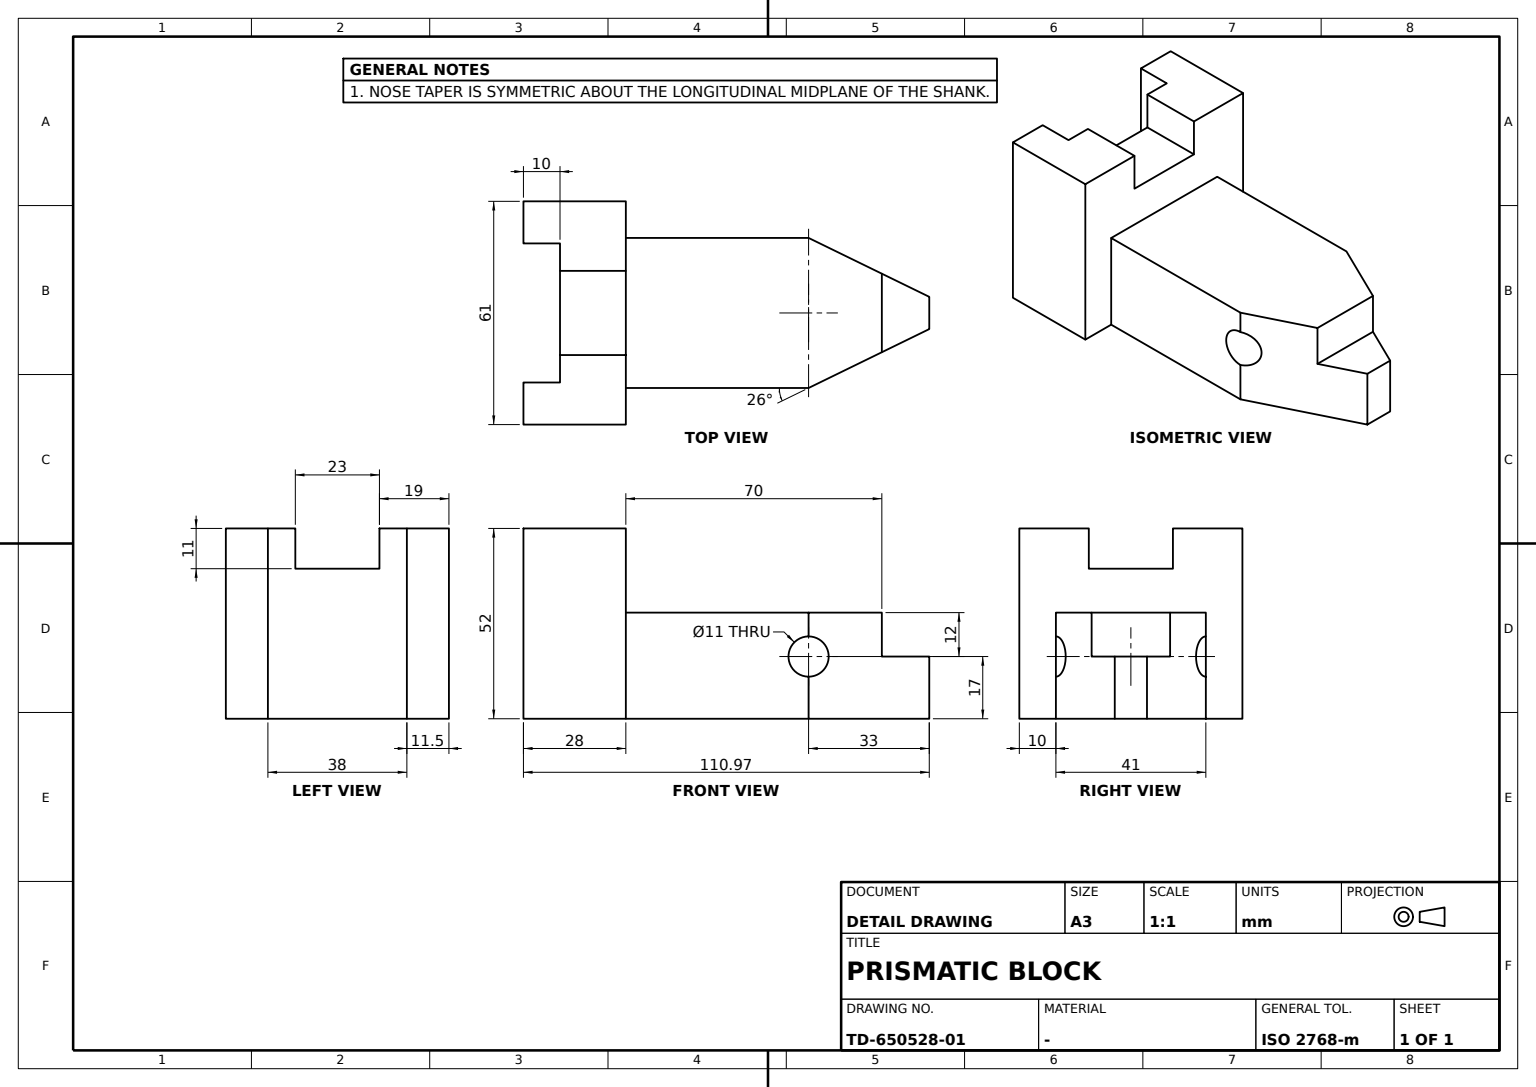
ISO-10303-21;
HEADER;
FILE_DESCRIPTION((''),'2;1');
FILE_NAME('','',(''),(''),'','','');
FILE_SCHEMA(('AUTOMOTIVE_DESIGN'));
ENDSEC;
DATA;
#1=APPLICATION_CONTEXT('');
#2=PRODUCT_CONTEXT('',#1,'mechanical');
#3=PRODUCT('','','',(#2));
#4=PRODUCT_DEFINITION_FORMATION('','',#3);
#5=PRODUCT_DEFINITION_CONTEXT('',#1,'design');
#6=PRODUCT_DEFINITION('','',#4,#5);
#7=PRODUCT_DEFINITION_SHAPE('','',#6);
#8=(LENGTH_UNIT()NAMED_UNIT(*)SI_UNIT(.MILLI.,.METRE.));
#9=(NAMED_UNIT(*)PLANE_ANGLE_UNIT()SI_UNIT($,.RADIAN.));
#10=(NAMED_UNIT(*)SI_UNIT($,.STERADIAN.)SOLID_ANGLE_UNIT());
#11=UNCERTAINTY_MEASURE_WITH_UNIT(LENGTH_MEASURE(0.005),#8,'distance_accuracy_value','');
#12=(GEOMETRIC_REPRESENTATION_CONTEXT(3)GLOBAL_UNCERTAINTY_ASSIGNED_CONTEXT((#11))GLOBAL_UNIT_ASSIGNED_CONTEXT((#8,#9,#10))REPRESENTATION_CONTEXT('',''));
#13=CARTESIAN_POINT('',(100.968771,-4.404825,0.));
#14=VERTEX_POINT('',#13);
#15=CARTESIAN_POINT('',(100.968771,4.404825,0.));
#16=VERTEX_POINT('',#15);
#17=DIRECTION('',(0.,1.,0.));
#18=VECTOR('',#17,1000.);
#19=LINE('',#13,#18);
#20=EDGE_CURVE('',#14,#16,#19,.T.);
#21=ORIENTED_EDGE('',*,*,#20,.T.);
#22=CARTESIAN_POINT('',(100.968771,4.404825,17.));
#23=VERTEX_POINT('',#22);
#24=DIRECTION('',(0.,0.,1.));
#25=VECTOR('',#24,1000.);
#26=LINE('',#15,#25);
#27=EDGE_CURVE('',#16,#23,#26,.T.);
#28=ORIENTED_EDGE('',*,*,#27,.T.);
#29=CARTESIAN_POINT('',(100.968771,-4.404825,17.));
#30=VERTEX_POINT('',#29);
#31=LINE('',#29,#18);
#32=EDGE_CURVE('',#30,#23,#31,.T.);
#33=ORIENTED_EDGE('',*,*,#32,.F.);
#34=LINE('',#13,#25);
#35=EDGE_CURVE('',#14,#30,#34,.T.);
#36=ORIENTED_EDGE('',*,*,#35,.F.);
#37=EDGE_LOOP('',(#21,#28,#33,#36));
#38=FACE_BOUND('',#37,.T.);
#39=DIRECTION('',(1.,0.,0.));
#40=DIRECTION('',(0.,0.,-1.));
#41=AXIS2_PLACEMENT_3D('',#13,#39,#40);
#42=PLANE('',#41);
#43=ADVANCED_FACE('',(#38),#42,.T.);
#44=CARTESIAN_POINT('',(-10.,-19.,0.));
#45=VERTEX_POINT('',#44);
#46=CARTESIAN_POINT('',(-10.,-30.5,0.));
#47=VERTEX_POINT('',#46);
#48=DIRECTION('',(0.,-1.,0.));
#49=VECTOR('',#48,1000.);
#50=LINE('',#44,#49);
#51=EDGE_CURVE('',#45,#47,#50,.T.);
#52=ORIENTED_EDGE('',*,*,#51,.T.);
#53=CARTESIAN_POINT('',(-10.,-30.5,52.));
#54=VERTEX_POINT('',#53);
#55=LINE('',#46,#25);
#56=EDGE_CURVE('',#47,#54,#55,.T.);
#57=ORIENTED_EDGE('',*,*,#56,.T.);
#58=CARTESIAN_POINT('',(-10.,-19.,52.));
#59=VERTEX_POINT('',#58);
#60=LINE('',#58,#49);
#61=EDGE_CURVE('',#59,#54,#60,.T.);
#62=ORIENTED_EDGE('',*,*,#61,.F.);
#63=LINE('',#44,#25);
#64=EDGE_CURVE('',#45,#59,#63,.T.);
#65=ORIENTED_EDGE('',*,*,#64,.F.);
#66=EDGE_LOOP('',(#52,#57,#62,#65));
#67=FACE_BOUND('',#66,.T.);
#68=DIRECTION('',(-1.,0.,0.));
#69=AXIS2_PLACEMENT_3D('',#44,#68,#48);
#70=PLANE('',#69);
#71=ADVANCED_FACE('',(#67),#70,.T.);
#72=CARTESIAN_POINT('',(0.,19.,0.));
#73=VERTEX_POINT('',#72);
#74=CARTESIAN_POINT('',(0.,19.,52.));
#75=VERTEX_POINT('',#74);
#76=LINE('',#72,#25);
#77=EDGE_CURVE('',#73,#75,#76,.T.);
#78=ORIENTED_EDGE('',*,*,#77,.T.);
#79=CARTESIAN_POINT('',(-10.,19.,52.));
#80=VERTEX_POINT('',#79);
#81=VECTOR('',#39,1000.);
#82=LINE('',#79,#81);
#83=EDGE_CURVE('',#80,#75,#82,.T.);
#84=ORIENTED_EDGE('',*,*,#83,.F.);
#85=CARTESIAN_POINT('',(-10.,19.,0.));
#86=VERTEX_POINT('',#85);
#87=LINE('',#85,#25);
#88=EDGE_CURVE('',#86,#80,#87,.T.);
#89=ORIENTED_EDGE('',*,*,#88,.F.);
#90=LINE('',#85,#81);
#91=EDGE_CURVE('',#86,#73,#90,.T.);
#92=ORIENTED_EDGE('',*,*,#91,.T.);
#93=EDGE_LOOP('',(#78,#84,#89,#92));
#94=FACE_BOUND('',#93,.T.);
#95=AXIS2_PLACEMENT_3D('',#85,#48,#40);
#96=PLANE('',#95);
#97=ADVANCED_FACE('',(#94),#96,.T.);
#98=ORIENTED_EDGE('',*,*,#64,.T.);
#99=CARTESIAN_POINT('',(0.,-19.,52.));
#100=VERTEX_POINT('',#99);
#101=VECTOR('',#68,1000.);
#102=LINE('',#99,#101);
#103=EDGE_CURVE('',#100,#59,#102,.T.);
#104=ORIENTED_EDGE('',*,*,#103,.F.);
#105=CARTESIAN_POINT('',(0.,-19.,0.));
#106=VERTEX_POINT('',#105);
#107=LINE('',#105,#25);
#108=EDGE_CURVE('',#106,#100,#107,.T.);
#109=ORIENTED_EDGE('',*,*,#108,.F.);
#110=LINE('',#105,#101);
#111=EDGE_CURVE('',#106,#45,#110,.T.);
#112=ORIENTED_EDGE('',*,*,#111,.T.);
#113=EDGE_LOOP('',(#98,#104,#109,#112));
#114=FACE_BOUND('',#113,.T.);
#115=AXIS2_PLACEMENT_3D('',#105,#17,#24);
#116=PLANE('',#115);
#117=ADVANCED_FACE('',(#114),#116,.T.);
#118=CARTESIAN_POINT('',(-10.,30.5,0.));
#119=VERTEX_POINT('',#118);
#120=LINE('',#118,#49);
#121=EDGE_CURVE('',#119,#86,#120,.T.);
#122=ORIENTED_EDGE('',*,*,#121,.T.);
#123=ORIENTED_EDGE('',*,*,#88,.T.);
#124=CARTESIAN_POINT('',(-10.,30.5,52.));
#125=VERTEX_POINT('',#124);
#126=LINE('',#124,#49);
#127=EDGE_CURVE('',#125,#80,#126,.T.);
#128=ORIENTED_EDGE('',*,*,#127,.F.);
#129=LINE('',#118,#25);
#130=EDGE_CURVE('',#119,#125,#129,.T.);
#131=ORIENTED_EDGE('',*,*,#130,.F.);
#132=EDGE_LOOP('',(#122,#123,#128,#131));
#133=FACE_BOUND('',#132,.T.);
#134=AXIS2_PLACEMENT_3D('',#118,#68,#24);
#135=PLANE('',#134);
#136=ADVANCED_FACE('',(#133),#135,.T.);
#137=CARTESIAN_POINT('',(18.,20.5,0.));
#138=VERTEX_POINT('',#137);
#139=CARTESIAN_POINT('',(18.,20.5,29.));
#140=VERTEX_POINT('',#139);
#141=LINE('',#137,#25);
#142=EDGE_CURVE('',#138,#140,#141,.T.);
#143=ORIENTED_EDGE('',*,*,#142,.F.);
#144=CARTESIAN_POINT('',(18.,30.5,0.));
#145=VERTEX_POINT('',#144);
#146=CARTESIAN_POINT('',(18.,-30.5,0.));
#147=LINE('',#146,#18);
#148=EDGE_CURVE('',#138,#145,#147,.T.);
#149=ORIENTED_EDGE('',*,*,#148,.T.);
#150=CARTESIAN_POINT('',(18.,30.5,52.));
#151=VERTEX_POINT('',#150);
#152=LINE('',#144,#25);
#153=EDGE_CURVE('',#145,#151,#152,.T.);
#154=ORIENTED_EDGE('',*,*,#153,.T.);
#155=CARTESIAN_POINT('',(18.,11.5,52.));
#156=VERTEX_POINT('',#155);
#157=CARTESIAN_POINT('',(18.,0.,52.));
#158=LINE('',#157,#18);
#159=EDGE_CURVE('',#156,#151,#158,.T.);
#160=ORIENTED_EDGE('',*,*,#159,.F.);
#161=CARTESIAN_POINT('',(18.,11.5,41.));
#162=VERTEX_POINT('',#161);
#163=VECTOR('',#40,1000.);
#164=LINE('',#155,#163);
#165=EDGE_CURVE('',#156,#162,#164,.T.);
#166=ORIENTED_EDGE('',*,*,#165,.T.);
#167=CARTESIAN_POINT('',(18.,-11.5,41.));
#168=VERTEX_POINT('',#167);
#169=LINE('',#167,#18);
#170=EDGE_CURVE('',#168,#162,#169,.T.);
#171=ORIENTED_EDGE('',*,*,#170,.F.);
#172=CARTESIAN_POINT('',(18.,-11.5,52.));
#173=VERTEX_POINT('',#172);
#174=LINE('',#172,#163);
#175=EDGE_CURVE('',#173,#168,#174,.T.);
#176=ORIENTED_EDGE('',*,*,#175,.F.);
#177=CARTESIAN_POINT('',(18.,-30.5,52.));
#178=VERTEX_POINT('',#177);
#179=EDGE_CURVE('',#178,#173,#158,.T.);
#180=ORIENTED_EDGE('',*,*,#179,.F.);
#181=VERTEX_POINT('',#146);
#182=LINE('',#146,#25);
#183=EDGE_CURVE('',#181,#178,#182,.T.);
#184=ORIENTED_EDGE('',*,*,#183,.F.);
#185=CARTESIAN_POINT('',(18.,-20.5,0.));
#186=VERTEX_POINT('',#185);
#187=EDGE_CURVE('',#181,#186,#147,.T.);
#188=ORIENTED_EDGE('',*,*,#187,.T.);
#189=CARTESIAN_POINT('',(18.,-20.5,29.));
#190=VERTEX_POINT('',#189);
#191=LINE('',#185,#25);
#192=EDGE_CURVE('',#186,#190,#191,.T.);
#193=ORIENTED_EDGE('',*,*,#192,.T.);
#194=LINE('',#139,#49);
#195=EDGE_CURVE('',#140,#190,#194,.T.);
#196=ORIENTED_EDGE('',*,*,#195,.F.);
#197=EDGE_LOOP('',(#143,#149,#154,#160,#166,#171,#176,#180,#184,#188,#193,#196));
#198=FACE_BOUND('',#197,.T.);
#199=CARTESIAN_POINT('',(18.,0.,0.));
#200=AXIS2_PLACEMENT_3D('',#199,#39,#40);
#201=PLANE('',#200);
#202=ADVANCED_FACE('',(#198),#201,.T.);
#203=CARTESIAN_POINT('',(0.,11.5,52.));
#204=VERTEX_POINT('',#203);
#205=CARTESIAN_POINT('',(0.,0.,52.));
#206=LINE('',#205,#49);
#207=EDGE_CURVE('',#75,#204,#206,.T.);
#208=ORIENTED_EDGE('',*,*,#207,.F.);
#209=ORIENTED_EDGE('',*,*,#77,.F.);
#210=LINE('',#72,#49);
#211=EDGE_CURVE('',#73,#106,#210,.T.);
#212=ORIENTED_EDGE('',*,*,#211,.T.);
#213=ORIENTED_EDGE('',*,*,#108,.T.);
#214=CARTESIAN_POINT('',(0.,-11.5,52.));
#215=VERTEX_POINT('',#214);
#216=EDGE_CURVE('',#215,#100,#206,.T.);
#217=ORIENTED_EDGE('',*,*,#216,.F.);
#218=CARTESIAN_POINT('',(0.,-11.5,41.));
#219=VERTEX_POINT('',#218);
#220=LINE('',#214,#163);
#221=EDGE_CURVE('',#215,#219,#220,.T.);
#222=ORIENTED_EDGE('',*,*,#221,.T.);
#223=CARTESIAN_POINT('',(0.,11.5,41.));
#224=VERTEX_POINT('',#223);
#225=LINE('',#223,#49);
#226=EDGE_CURVE('',#224,#219,#225,.T.);
#227=ORIENTED_EDGE('',*,*,#226,.F.);
#228=LINE('',#203,#163);
#229=EDGE_CURVE('',#204,#224,#228,.T.);
#230=ORIENTED_EDGE('',*,*,#229,.F.);
#231=EDGE_LOOP('',(#208,#209,#212,#213,#217,#222,#227,#230));
#232=FACE_BOUND('',#231,.T.);
#233=CARTESIAN_POINT('',(0.,0.,0.));
#234=AXIS2_PLACEMENT_3D('',#233,#68,#48);
#235=PLANE('',#234);
#236=ADVANCED_FACE('',(#232),#235,.T.);
#237=CARTESIAN_POINT('',(67.968771,-20.5,22.5));
#238=VERTEX_POINT('',#237);
#239=CARTESIAN_POINT('',(67.968771,20.5,22.5));
#240=VERTEX_POINT('',#239);
#241=CARTESIAN_POINT('',(67.968771,-30.,22.5));
#242=LINE('',#241,#18);
#243=EDGE_CURVE('',#238,#240,#242,.T.);
#244=ORIENTED_EDGE('',*,*,#243,.F.);
#245=CARTESIAN_POINT('',(67.968771,-20.5,11.5));
#246=VERTEX_POINT('',#245);
#247=CARTESIAN_POINT('',(67.968771,-20.5,17.));
#248=AXIS2_PLACEMENT_3D('',#247,#17,#39);
#249=CIRCLE('',#248,5.5);
#250=EDGE_CURVE('',#246,#238,#249,.T.);
#251=ORIENTED_EDGE('',*,*,#250,.F.);
#252=CARTESIAN_POINT('',(67.968771,20.5,11.5));
#253=VERTEX_POINT('',#252);
#254=CARTESIAN_POINT('',(67.968771,-30.,11.5));
#255=LINE('',#254,#18);
#256=EDGE_CURVE('',#253,#246,#255,.F.);
#257=ORIENTED_EDGE('',*,*,#256,.F.);
#258=CARTESIAN_POINT('',(67.968771,20.5,17.));
#259=AXIS2_PLACEMENT_3D('',#258,#48,#68);
#260=CIRCLE('',#259,5.5);
#261=EDGE_CURVE('',#240,#253,#260,.T.);
#262=ORIENTED_EDGE('',*,*,#261,.F.);
#263=EDGE_LOOP('',(#244,#251,#257,#262));
#264=FACE_BOUND('',#263,.T.);
#265=CARTESIAN_POINT('',(67.968771,-30.,17.));
#266=AXIS2_PLACEMENT_3D('',#265,#17,#24);
#267=CYLINDRICAL_SURFACE('',#266,5.5);
#268=ADVANCED_FACE('',(#264),#267,.F.);
#269=LINE('',#53,#81);
#270=EDGE_CURVE('',#54,#178,#269,.T.);
#271=ORIENTED_EDGE('',*,*,#270,.T.);
#272=ORIENTED_EDGE('',*,*,#179,.T.);
#273=LINE('',#214,#81);
#274=EDGE_CURVE('',#215,#173,#273,.T.);
#275=ORIENTED_EDGE('',*,*,#274,.F.);
#276=ORIENTED_EDGE('',*,*,#216,.T.);
#277=ORIENTED_EDGE('',*,*,#103,.T.);
#278=ORIENTED_EDGE('',*,*,#61,.T.);
#279=EDGE_LOOP('',(#271,#272,#275,#276,#277,#278));
#280=FACE_BOUND('',#279,.T.);
#281=AXIS2_PLACEMENT_3D('',#205,#24,#39);
#282=PLANE('',#281);
#283=ADVANCED_FACE('',(#280),#282,.T.);
#284=CARTESIAN_POINT('',(88.,-10.730117,29.));
#285=VERTEX_POINT('',#284);
#286=CARTESIAN_POINT('',(88.,-10.730117,17.));
#287=VERTEX_POINT('',#286);
#288=LINE('',#284,#163);
#289=EDGE_CURVE('',#285,#287,#288,.T.);
#290=ORIENTED_EDGE('',*,*,#289,.T.);
#291=CARTESIAN_POINT('',(88.,10.730117,17.));
#292=VERTEX_POINT('',#291);
#293=LINE('',#291,#18);
#294=EDGE_CURVE('',#287,#292,#293,.T.);
#295=ORIENTED_EDGE('',*,*,#294,.T.);
#296=CARTESIAN_POINT('',(88.,10.730117,29.));
#297=VERTEX_POINT('',#296);
#298=LINE('',#296,#163);
#299=EDGE_CURVE('',#297,#292,#298,.T.);
#300=ORIENTED_EDGE('',*,*,#299,.F.);
#301=LINE('',#296,#49);
#302=EDGE_CURVE('',#297,#285,#301,.T.);
#303=ORIENTED_EDGE('',*,*,#302,.T.);
#304=EDGE_LOOP('',(#290,#295,#300,#303));
#305=FACE_BOUND('',#304,.T.);
#306=AXIS2_PLACEMENT_3D('',#296,#39,#17);
#307=PLANE('',#306);
#308=ADVANCED_FACE('',(#305),#307,.T.);
#309=ORIENTED_EDGE('',*,*,#187,.F.);
#310=LINE('',#46,#81);
#311=EDGE_CURVE('',#47,#181,#310,.T.);
#312=ORIENTED_EDGE('',*,*,#311,.F.);
#313=ORIENTED_EDGE('',*,*,#51,.F.);
#314=ORIENTED_EDGE('',*,*,#111,.F.);
#315=ORIENTED_EDGE('',*,*,#211,.F.);
#316=ORIENTED_EDGE('',*,*,#91,.F.);
#317=ORIENTED_EDGE('',*,*,#121,.F.);
#318=LINE('',#144,#101);
#319=EDGE_CURVE('',#145,#119,#318,.T.);
#320=ORIENTED_EDGE('',*,*,#319,.F.);
#321=ORIENTED_EDGE('',*,*,#148,.F.);
#322=CARTESIAN_POINT('',(67.968771,20.5,0.));
#323=VERTEX_POINT('',#322);
#324=LINE('',#322,#101);
#325=EDGE_CURVE('',#323,#138,#324,.T.);
#326=ORIENTED_EDGE('',*,*,#325,.F.);
#327=DIRECTION('',(-0.898794046,0.438371147,0.));
#328=VECTOR('',#327,1000.);
#329=LINE('',#15,#328);
#330=EDGE_CURVE('',#16,#323,#329,.T.);
#331=ORIENTED_EDGE('',*,*,#330,.F.);
#332=ORIENTED_EDGE('',*,*,#20,.F.);
#333=CARTESIAN_POINT('',(67.968771,-20.5,0.));
#334=VERTEX_POINT('',#333);
#335=DIRECTION('',(0.898794046,0.438371147,0.));
#336=VECTOR('',#335,1000.);
#337=LINE('',#333,#336);
#338=EDGE_CURVE('',#334,#14,#337,.T.);
#339=ORIENTED_EDGE('',*,*,#338,.F.);
#340=LINE('',#185,#81);
#341=EDGE_CURVE('',#186,#334,#340,.T.);
#342=ORIENTED_EDGE('',*,*,#341,.F.);
#343=EDGE_LOOP('',(#309,#312,#313,#314,#315,#316,#317,#320,#321,#326,#331,#332,#339,#342));
#344=FACE_BOUND('',#343,.T.);
#345=AXIS2_PLACEMENT_3D('',#233,#24,#39);
#346=PLANE('',#345);
#347=ADVANCED_FACE('',(#344),#346,.F.);
#348=ORIENTED_EDGE('',*,*,#229,.T.);
#349=LINE('',#161,#81);
#350=EDGE_CURVE('',#224,#162,#349,.T.);
#351=ORIENTED_EDGE('',*,*,#350,.T.);
#352=ORIENTED_EDGE('',*,*,#165,.F.);
#353=LINE('',#155,#101);
#354=EDGE_CURVE('',#156,#204,#353,.T.);
#355=ORIENTED_EDGE('',*,*,#354,.T.);
#356=EDGE_LOOP('',(#348,#351,#352,#355));
#357=FACE_BOUND('',#356,.T.);
#358=AXIS2_PLACEMENT_3D('',#155,#48,#39);
#359=PLANE('',#358);
#360=ADVANCED_FACE('',(#357),#359,.T.);
#361=ORIENTED_EDGE('',*,*,#243,.T.);
#362=CARTESIAN_POINT('',(78.968771,15.134942,11.5));
#363=CARTESIAN_POINT('',(78.968771,15.134942,22.5));
#364=(BOUNDED_CURVE()B_SPLINE_CURVE(3,(#252,#362,#363,#239),.UNSPECIFIED.,.F.,.F.)B_SPLINE_CURVE_WITH_KNOTS((4,4),(1.570796327,4.71238898),.UNSPECIFIED.)CURVE()GEOMETRIC_REPRESENTATION_ITEM()RATIONAL_B_SPLINE_CURVE((1.,0.333333333,0.333333333,1.))REPRESENTATION_ITEM(''));
#365=EDGE_CURVE('',#253,#240,#364,.T.);
#366=ORIENTED_EDGE('',*,*,#365,.F.);
#367=ORIENTED_EDGE('',*,*,#256,.T.);
#368=CARTESIAN_POINT('',(78.968771,-15.134942,22.5));
#369=CARTESIAN_POINT('',(78.968771,-15.134942,11.5));
#370=(BOUNDED_CURVE()B_SPLINE_CURVE(3,(#237,#368,#369,#245),.UNSPECIFIED.,.F.,.F.)B_SPLINE_CURVE_WITH_KNOTS((4,4),(4.71238898,7.853981634),.UNSPECIFIED.)CURVE()GEOMETRIC_REPRESENTATION_ITEM()RATIONAL_B_SPLINE_CURVE((1.,0.333333333,0.333333333,1.))REPRESENTATION_ITEM(''));
#371=EDGE_CURVE('',#238,#246,#370,.T.);
#372=ORIENTED_EDGE('',*,*,#371,.F.);
#373=EDGE_LOOP('',(#361,#366,#367,#372));
#374=FACE_BOUND('',#373,.T.);
#375=ADVANCED_FACE('',(#374),#267,.F.);
#376=CARTESIAN_POINT('',(67.968771,20.5,29.));
#377=VERTEX_POINT('',#376);
#378=LINE('',#376,#101);
#379=EDGE_CURVE('',#377,#140,#378,.T.);
#380=ORIENTED_EDGE('',*,*,#379,.T.);
#381=ORIENTED_EDGE('',*,*,#195,.T.);
#382=CARTESIAN_POINT('',(67.968771,-20.5,29.));
#383=VERTEX_POINT('',#382);
#384=LINE('',#189,#81);
#385=EDGE_CURVE('',#190,#383,#384,.T.);
#386=ORIENTED_EDGE('',*,*,#385,.T.);
#387=LINE('',#382,#336);
#388=EDGE_CURVE('',#383,#285,#387,.T.);
#389=ORIENTED_EDGE('',*,*,#388,.T.);
#390=ORIENTED_EDGE('',*,*,#302,.F.);
#391=CARTESIAN_POINT('',(100.968771,4.404825,29.));
#392=LINE('',#391,#328);
#393=EDGE_CURVE('',#297,#377,#392,.T.);
#394=ORIENTED_EDGE('',*,*,#393,.T.);
#395=EDGE_LOOP('',(#380,#381,#386,#389,#390,#394));
#396=FACE_BOUND('',#395,.T.);
#397=CARTESIAN_POINT('',(0.,0.,29.));
#398=AXIS2_PLACEMENT_3D('',#397,#24,#39);
#399=PLANE('',#398);
#400=ADVANCED_FACE('',(#396),#399,.T.);
#401=ORIENTED_EDGE('',*,*,#175,.T.);
#402=LINE('',#218,#101);
#403=EDGE_CURVE('',#168,#219,#402,.T.);
#404=ORIENTED_EDGE('',*,*,#403,.T.);
#405=ORIENTED_EDGE('',*,*,#221,.F.);
#406=ORIENTED_EDGE('',*,*,#274,.T.);
#407=EDGE_LOOP('',(#401,#404,#405,#406));
#408=FACE_BOUND('',#407,.T.);
#409=AXIS2_PLACEMENT_3D('',#214,#17,#68);
#410=PLANE('',#409);
#411=ADVANCED_FACE('',(#408),#410,.T.);
#412=ORIENTED_EDGE('',*,*,#226,.T.);
#413=ORIENTED_EDGE('',*,*,#403,.F.);
#414=ORIENTED_EDGE('',*,*,#170,.T.);
#415=ORIENTED_EDGE('',*,*,#350,.F.);
#416=EDGE_LOOP('',(#412,#413,#414,#415));
#417=FACE_BOUND('',#416,.T.);
#418=CARTESIAN_POINT('',(0.,0.,41.));
#419=AXIS2_PLACEMENT_3D('',#418,#24,#39);
#420=PLANE('',#419);
#421=ADVANCED_FACE('',(#417),#420,.T.);
#422=LINE('',#333,#25);
#423=EDGE_CURVE('',#238,#383,#422,.T.);
#424=ORIENTED_EDGE('',*,*,#423,.T.);
#425=ORIENTED_EDGE('',*,*,#385,.F.);
#426=ORIENTED_EDGE('',*,*,#192,.F.);
#427=ORIENTED_EDGE('',*,*,#341,.T.);
#428=EDGE_CURVE('',#334,#246,#422,.T.);
#429=ORIENTED_EDGE('',*,*,#428,.T.);
#430=ORIENTED_EDGE('',*,*,#250,.T.);
#431=EDGE_LOOP('',(#424,#425,#426,#427,#429,#430));
#432=FACE_BOUND('',#431,.T.);
#433=AXIS2_PLACEMENT_3D('',#185,#48,#39);
#434=PLANE('',#433);
#435=ADVANCED_FACE('',(#432),#434,.T.);
#436=ORIENTED_EDGE('',*,*,#159,.T.);
#437=LINE('',#150,#101);
#438=EDGE_CURVE('',#151,#125,#437,.T.);
#439=ORIENTED_EDGE('',*,*,#438,.T.);
#440=ORIENTED_EDGE('',*,*,#127,.T.);
#441=ORIENTED_EDGE('',*,*,#83,.T.);
#442=ORIENTED_EDGE('',*,*,#207,.T.);
#443=ORIENTED_EDGE('',*,*,#354,.F.);
#444=EDGE_LOOP('',(#436,#439,#440,#441,#442,#443));
#445=FACE_BOUND('',#444,.T.);
#446=ADVANCED_FACE('',(#445),#282,.T.);
#447=ORIENTED_EDGE('',*,*,#27,.F.);
#448=ORIENTED_EDGE('',*,*,#330,.T.);
#449=LINE('',#322,#25);
#450=EDGE_CURVE('',#323,#253,#449,.T.);
#451=ORIENTED_EDGE('',*,*,#450,.T.);
#452=ORIENTED_EDGE('',*,*,#365,.T.);
#453=EDGE_CURVE('',#240,#377,#449,.T.);
#454=ORIENTED_EDGE('',*,*,#453,.T.);
#455=ORIENTED_EDGE('',*,*,#393,.F.);
#456=ORIENTED_EDGE('',*,*,#299,.T.);
#457=LINE('',#22,#328);
#458=EDGE_CURVE('',#23,#292,#457,.T.);
#459=ORIENTED_EDGE('',*,*,#458,.F.);
#460=EDGE_LOOP('',(#447,#448,#451,#452,#454,#455,#456,#459));
#461=FACE_BOUND('',#460,.T.);
#462=DIRECTION('',(0.438371147,0.898794046,0.));
#463=AXIS2_PLACEMENT_3D('',#15,#462,#327);
#464=PLANE('',#463);
#465=ADVANCED_FACE('',(#461),#464,.T.);
#466=ORIENTED_EDGE('',*,*,#270,.F.);
#467=ORIENTED_EDGE('',*,*,#56,.F.);
#468=ORIENTED_EDGE('',*,*,#311,.T.);
#469=ORIENTED_EDGE('',*,*,#183,.T.);
#470=EDGE_LOOP('',(#466,#467,#468,#469));
#471=FACE_BOUND('',#470,.T.);
#472=AXIS2_PLACEMENT_3D('',#46,#48,#40);
#473=PLANE('',#472);
#474=ADVANCED_FACE('',(#471),#473,.T.);
#475=ORIENTED_EDGE('',*,*,#35,.T.);
#476=LINE('',#286,#336);
#477=EDGE_CURVE('',#287,#30,#476,.T.);
#478=ORIENTED_EDGE('',*,*,#477,.F.);
#479=ORIENTED_EDGE('',*,*,#289,.F.);
#480=ORIENTED_EDGE('',*,*,#388,.F.);
#481=ORIENTED_EDGE('',*,*,#423,.F.);
#482=ORIENTED_EDGE('',*,*,#371,.T.);
#483=ORIENTED_EDGE('',*,*,#428,.F.);
#484=ORIENTED_EDGE('',*,*,#338,.T.);
#485=EDGE_LOOP('',(#475,#478,#479,#480,#481,#482,#483,#484));
#486=FACE_BOUND('',#485,.T.);
#487=DIRECTION('',(0.438371147,-0.898794046,0.));
#488=AXIS2_PLACEMENT_3D('',#333,#487,#335);
#489=PLANE('',#488);
#490=ADVANCED_FACE('',(#486),#489,.T.);
#491=ORIENTED_EDGE('',*,*,#319,.T.);
#492=ORIENTED_EDGE('',*,*,#130,.T.);
#493=ORIENTED_EDGE('',*,*,#438,.F.);
#494=ORIENTED_EDGE('',*,*,#153,.F.);
#495=EDGE_LOOP('',(#491,#492,#493,#494));
#496=FACE_BOUND('',#495,.T.);
#497=AXIS2_PLACEMENT_3D('',#144,#17,#24);
#498=PLANE('',#497);
#499=ADVANCED_FACE('',(#496),#498,.T.);
#500=ORIENTED_EDGE('',*,*,#458,.T.);
#501=ORIENTED_EDGE('',*,*,#294,.F.);
#502=ORIENTED_EDGE('',*,*,#477,.T.);
#503=ORIENTED_EDGE('',*,*,#32,.T.);
#504=EDGE_LOOP('',(#500,#501,#502,#503));
#505=FACE_BOUND('',#504,.T.);
#506=CARTESIAN_POINT('',(0.,0.,17.));
#507=AXIS2_PLACEMENT_3D('',#506,#24,#39);
#508=PLANE('',#507);
#509=ADVANCED_FACE('',(#505),#508,.T.);
#510=ORIENTED_EDGE('',*,*,#450,.F.);
#511=ORIENTED_EDGE('',*,*,#325,.T.);
#512=ORIENTED_EDGE('',*,*,#142,.T.);
#513=ORIENTED_EDGE('',*,*,#379,.F.);
#514=ORIENTED_EDGE('',*,*,#453,.F.);
#515=ORIENTED_EDGE('',*,*,#261,.T.);
#516=EDGE_LOOP('',(#510,#511,#512,#513,#514,#515));
#517=FACE_BOUND('',#516,.T.);
#518=AXIS2_PLACEMENT_3D('',#322,#17,#68);
#519=PLANE('',#518);
#520=ADVANCED_FACE('',(#517),#519,.T.);
#521=CLOSED_SHELL('',(#43,#71,#97,#117,#136,#202,#236,#268,#283,#308,#347,#360,#375,#400,#411,#421,#435,#446,#465,#474,#490,#499,#509,#520));
#522=MANIFOLD_SOLID_BREP('',#521);
#523=ADVANCED_BREP_SHAPE_REPRESENTATION('',(#522),#12);
#524=SHAPE_DEFINITION_REPRESENTATION(#7,#523);
ENDSEC;
END-ISO-10303-21;
